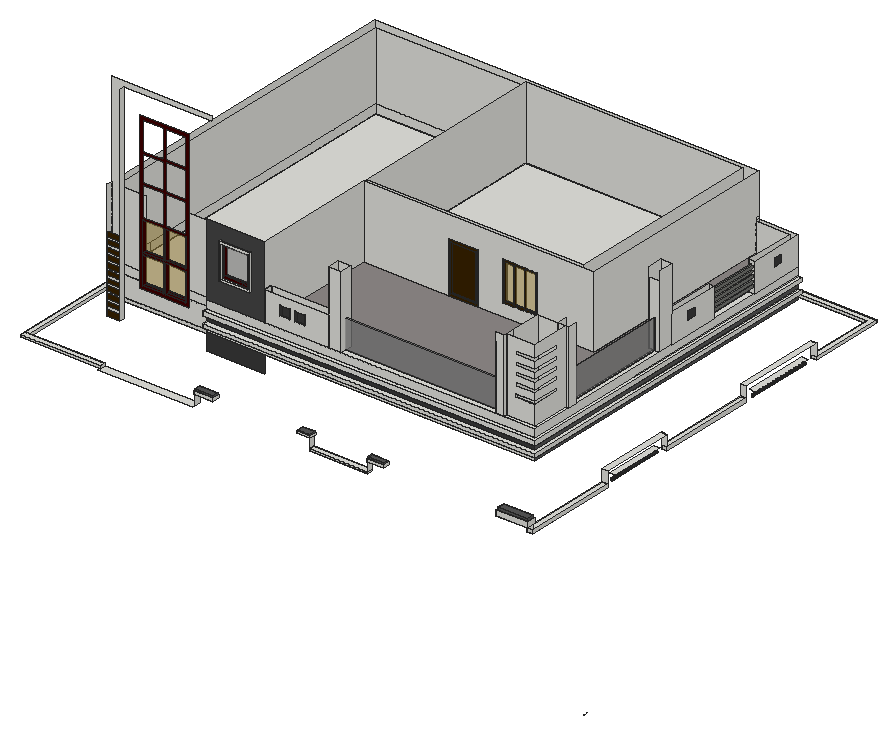
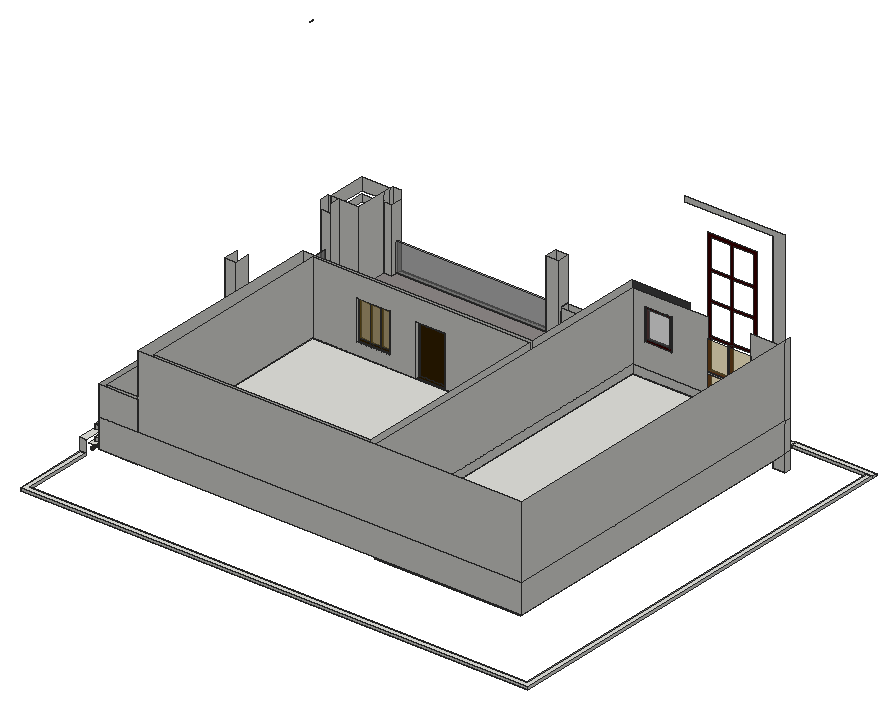
# SketchUp Ruby script. Lengths in inches.
U = 1.inch
M = Sketchup.active_model
def pt(a) = Geom::Point3d.new(a.map { |v| v * U })
def face(e, loops, mat)
  f = e.add_face(loops[0].map { |a| pt(a) })
  loops[1..].each { |l| e.add_face(l.map { |a| pt(a) }).erase! }
  f.material = f.back_material = mat if mat
  f
end
# faces: each face lists its corners as indices into pts; further lists are holes
def faces(e, pts, list, mat = nil) = list.each { |f| face(e, (f[0].is_a?(Array) ? f : [f]).map { |l| l.map { |i| pts[i] } }, mat) }
# xy, xz, yz: faces in a plane at the given z, y or x. An outline is a flat list of corners, or four numbers for a rectangle; further outlines are holes
def ring(l) = l.size == 4 ? [[l[0], l[1]], [l[2], l[1]], [l[2], l[3]], [l[0], l[3]]] : l.each_slice(2).to_a
def flat(e, list, mat, &to3) = list.each { |f| face(e, (f[0].is_a?(Array) ? f : [f]).map { |l| ring(l).map { |u, v| to3.(u, v) } }, mat) }
def xy(e, z, list, mat = nil) = flat(e, list, mat) { |x, y| [x, y, z] }
def xz(e, y, list, mat = nil) = flat(e, list, mat) { |x, z| [x, y, z] }
def yz(e, x, list, mat = nil) = flat(e, list, mat) { |y, z| [x, y, z] }
def lines(e, pts, list) = list.each { |a, b| e.add_line(pt(pts[a]), pt(pts[b])) }
# prism: a flat outline (further loops are holes) pulled along v
def prism(e, loops, v, mat = nil)
  f = face(e, loops, mat); d = Geom::Vector3d.new(v.map { |x| x * U })
  f.pushpull(f.normal.samedirection?(d) ? d.length : -d.length)
end
def box(e, o, s, mat = nil) = prism(e, [[o, [o[0] + s[0], o[1], o[2]], [o[0] + s[0], o[1] + s[1], o[2]], [o[0], o[1] + s[1], o[2]]]], [0, 0, s[2]], mat)
def at(x, y, z, deg = 0) = Geom::Transformation.translation(pt([x, y, z])) * Geom::Transformation.rotation(ORIGIN, Z_AXIS, deg.degrees)
def axes(o, x, y, z) = Geom::Transformation.new([*x, 0, *y, 0, *z, 0, *pt(o).to_a, 1])
def part(name) = M.definitions.add(name)
# library, detail: a bought-in or finely detailed component or shape, given as its bounding box
def library(name, o, s) = part(name).tap { |d| box(d.entities, o, s) }
def detail(e, o, s) = box(e.add_group.entities, o, s)
def put(e, d, t, mat = nil) = e.add_instance(d, t).tap { |i| i.material = mat if mat }
def group(e, t, mat = nil) = e.add_group.tap { |g| g.transformation = t; g.material = mat if mat }.entities
root = M.entities
M.materials.add("[Color A08]").color = [56, 34, 0]
M.materials.add("[Color A08]1").color = [63, 0, 0]
M.materials.add("[Color M06]").color = [86, 86, 86]
M.materials.add("[Color M07]").color = [58, 58, 58]
M.materials.add("[Color M08]").color = [30, 30, 30]
M.materials.add("[Granite Dark Gray]").color = [69, 68, 68]
M.materials.add("[Metal Seamed]1").color = [118, 119, 115]
M.materials.add("[Stone Marble]").color = [143, 138, 136]
M.materials.add("[Translucent Glass Blue]").color = [179, 149, 61]
M.materials["[Translucent Glass Blue]"].alpha = 0.5
M.materials.add("[Translucent Glass Gray]").color = [128, 128, 128]
M.materials["[Translucent Glass Gray]"].alpha = 0.5
c1 = part("Group\#1")
xy(c1.entities,0,[[0,0,48,2.75]],"[Color A08]")
xy(c1.entities,3.37,[[3.37,0,44.63,2.75]],"[Color A08]")
xy(c1.entities,80.63,[[3.37,0,44.63,2.75]],"[Color A08]")
xy(c1.entities,84,[[0,0,48,2.75]],"[Color A08]")
xz(c1.entities,0,[[[0,0,48,84],[3.37,3.37,44.63,80.63]]],"[Color A08]")
xz(c1.entities,2.75,[[[0,0,48,84],[3.37,3.37,44.63,80.63]],[3.37,3.37,44.63,80.63]],"[Color A08]")
yz(c1.entities,0,[[0,0,2.75,84]],"[Color A08]")
yz(c1.entities,3.37,[[0,3.37,2.75,80.63]],"[Color A08]")
yz(c1.entities,44.63,[[0,3.37,2.75,80.63]],"[Color A08]")
yz(c1.entities,48,[[0,0,2.75,84]],"[Color A08]")
c2 = part("Group\#2")
xy(c2.entities,0,[[0,0,80.25,5.625]],"[Color A08]")
xy(c2.entities,3.1,[[3.1,0,25.78,5.625],[27.03,0,50.28,5.625],[51.53,0,77.15,5.625]],"[Color A08]")
xy(c2.entities,66.65,[[3.1,0,25.78,5.625],[27.03,0,50.28,5.625],[51.53,0,77.15,5.625]],"[Color A08]")
xy(c2.entities,69.75,[[0,0,80.25,5.625]],"[Color A08]")
xz(c2.entities,0,[[[0,0,80.25,69.75],[51.53,3.1,77.15,66.65],[27.03,3.1,50.28,66.65],[3.1,3.1,25.78,66.65]]],"[Color A08]")
xz(c2.entities,5.625,[[[0,0,80.25,69.75],[51.53,3.1,77.15,66.65],[27.03,3.1,50.28,66.65],[3.1,3.1,25.78,66.65]]],"[Color A08]")
xz(c2.entities,5.625,[[3.1,3.1,25.78,66.65],[27.03,3.1,50.28,66.65],[51.53,3.1,77.15,66.65]],"[Translucent Glass Blue]")
yz(c2.entities,0,[[0,0,5.625,69.75]],"[Color A08]")
yz(c2.entities,3.1,[[0,3.1,5.625,66.65]],"[Color A08]")
yz(c2.entities,25.78,[[0,3.1,5.625,66.65]],"[Color A08]")
yz(c2.entities,27.03,[[0,3.1,5.625,66.65]],"[Color A08]")
yz(c2.entities,50.28,[[0,3.1,5.625,66.65]],"[Color A08]")
yz(c2.entities,51.53,[[0,3.1,5.625,66.65]],"[Color A08]")
yz(c2.entities,77.15,[[0,3.1,5.625,66.65]],"[Color A08]")
yz(c2.entities,80.25,[[0,0,5.625,69.75]],"[Color A08]")
prism(root,[[[834.64,582.45,107.43],[835.13,582.45,107.31],[835.64,582.45,107.32],[836.12,582.45,107.46],[836.55,582.45,107.73],[836.9,582.45,108.09],[837.14,582.45,108.54],[837.26,582.45,109.03],[837.25,582.45,109.53],[837.11,582.45,110.02],[836.85,582.45,110.45],[836.48,582.45,110.8],[836.04,582.45,111.04],[835.55,582.45,111.16],[835.04,582.45,111.15],[834.55,582.45,111.01],[834.12,582.45,110.74],[833.77,582.45,110.38],[833.53,582.45,109.93],[833.41,582.45,109.44],[833.42,582.45,108.9375],[833.57,582.45,108.45],[833.83,582.45,108.02],[834.19,582.45,107.67]]],[0,91.75,0],"[Color M07]")
xy(root,105,[[132.5,398.15,288.93,411.9],[0,402.9,132.5,411.9],[478.28,402.9,575.03,411.9],[0,411.9,0,1122.9,840,1122.9,840,999.11,831,999.11,831,1113.9,9,1113.9,9,411.9],[831,411.9,840,566.77],
  [831,690.36,840,853.98]])
xy(root,107.75,[[478.28,402.9,575.03,411.9]])
xy(root,109,[[0,402.9,132.5,411.9],[0,411.9,9,411.9,9,1113.9,831,1113.9,831,999.11,840,999.11,840,1122.9,0,1122.9]])
xy(root,110.5,[[831,411.9,840,566.77]])
xy(root,111.25,[[831,690.36,840,853.98]])
xy(root,113.38,[[831,872.22,840,980.28]])
xy(root,117,[[470.84,700.96,518.84,706.96]])
xy(root,117.03,[[831,582.45,840,674.33]])
xy(root,119.375,[[789.41,399.71,789.41,415.09,831,415.09,831,411.9,791.47,411.9,791.47,402.9,840,402.9,840,411.9,831,411.9,831,415.09,841.625,415.09,841.625,399.71]])
xy(root,122.6875,[[[287.74,401.21,319.84,413.9],[288.93,402.9,318.78,411.9]]])
xy(root,122.82,[[560.85,700.96,616.42,706.96]])
xy(root,123,[[791.47,402.9,840,411.9]])
xy(root,123.125,[[[574.09,401.34,602.04,413.34],[575.03,402.9,600.6,411.9]]])
xy(root,124.5625,[[288.93,402.9,318.78,411.9]])
xy(root,124.6875,[[[458.12,401.02,479.97,413.09],[459.31,402.9,478.28,411.9]]])
xy(root,124.8125,[[575.03,402.9,600.6,411.9]])
xy(root,125.23,[[75.5,487.84,96.69,496.71]])
xy(root,125.4375,[[459.31,402.9,478.28,411.9]])
xy(root,127.5625,[[[789.41,399.71,841.625,415.09],[791.47,401.77,840,413.15]],[[458.12,401.02,479.97,413.09],[458.93,402.02,479.22,412.65]],[[287.74,401.21,319.84,413.9],[288.43,402.46,318.78,412.77]],[[574.09,401.34,602.04,413.34],[575.03,402.59,600.85,411.96]],[791.47,401.77,840,413.15],
  [458.93,402.02,479.22,412.65],[288.43,402.46,318.78,412.77],[575.03,402.59,600.85,411.96]])
xy(root,129.375,[[575.03,402.59,600.85,411.96]],"[Color M06]")
xy(root,129.5,[[831,566.77,840,690.36],[831,853.98,840,999.11]])
xy(root,129.5,[[458.93,402.02,479.22,412.65]],"[Color M06]")
xy(root,130,[[288.43,402.46,318.78,412.77]],"[Color M06]")
xy(root,131.6875,[[791.47,401.77,840,413.15]],"[Color M06]")
xy(root,147,[[81.5,502.71,323.75,1035.15]])
xy(root,153,[[329.75,496.71,329.75,700.96,710.3125,700.96,710.3125,1041.15,776.3125,1041.15,776.3125,496.71],[81.5,502.71,323.75,1035.15]])
xy(root,163.0625,[[233.4,489.27,329.75,496.71],[329.75,489.27,782.0625,496.71],[329.75,496.71,776.3125,700.96],[776.3125,496.71,782.0625,1041.09]])
xy(root,163.22,[[1254.01,0,1254.88,6]],"[Color M08]")
xy(root,169.125,[[233.4,489.27,782.0625,489.27,782.0625,1041.09,776.3125,1041.09,776.3125,496.71,233.4,496.71],[329.75,496.71,776.3125,700.96]])
xy(root,180.8125,[[233.4,489.27,329.75,496.71],[329.75,489.27,782.0625,496.71],[329.75,496.71,776.3125,700.96],[776.3125,496.71,782.0625,1041.15]])
xy(root,184.79,[[128.05,496.71,161.69,502.71],[165.04,496.71,198.99,502.71]],"[Color A08]1")
xy(root,187,[[81.5,502.71,323.75,1035.15]])
xy(root,187.875,[[233.4,489.27,782.0625,489.27,782.0625,1041.15,776.3125,1041.15,776.3125,496.71,233.4,496.71],[329.75,496.71,776.3125,700.96]])
xy(root,195,[[329.75,706.96,689.4375,1035.15]])
xy(root,201,[[329.75,496.71,434.48,511.31],[434.48,496.71,455.35,516.84],[455.35,496.71,712.1,504.34],[712.1,496.71,724.73,514.59],[724.73,496.71,776.3125,502.4],
  [724.73,502.4,771.75,566.61],[771.75,502.4,776.3125,566.61],[455.35,504.34,712.1,506.34],[758.97,566.61,776.3125,581.49],[767.0625,581.49,769.0625,754.59],
  [769.0625,581.49,776.3125,754.59],[329.75,706.96,689.4375,1035.15],[689.4375,706.96,710.3125,1035.15],[758.0625,754.59,776.3125,780.03],[767.1875,780.03,776.3125,867.13],
  [767.1875,867.13,776.3125,951.14],[767.1875,951.14,767.1875,1035.15,710.3125,1035.15,710.3125,1041.15,776.3125,1041.15,776.3125,951.14]])
xy(root,201,[[455.35,506.34,712.1,506.34,712.1,514.59,724.73,514.59,724.73,566.61,758.97,566.61,758.97,581.49,767.0625,581.49,767.0625,754.59,758.0625,754.59,758.0625,780.03,767.1875,780.03,767.1875,1035.15,710.3125,1035.15,710.3125,700.96,518.51,700.96,518.51,706.96,470.51,706.96,470.51,700.96,329.75,700.96,329.75,511.31,434.48,511.31,434.48,516.84,455.35,516.84]],"[Stone Marble]")
xy(root,208.99,[[769.27,867.13,773.7,951.14]],"[Metal Seamed]1")
xy(root,212.93,[[769.27,867.13,773.7,951.14]],"[Metal Seamed]1")
xy(root,216.37,[[769.27,867.13,773.7,952.63]],"[Metal Seamed]1")
xy(root,219.98,[[354.55,496.71,370.43,499.46],[379.61,496.71,395.49,499.46]],"[Color M07]")
xy(root,220.31,[[769.27,867.13,773.7,952.63]],"[Metal Seamed]1")
xy(root,221.54,[[773.75,811.33,776.3125,829.45],[773.3125,989.77,776.3125,1007.89]],"[Color M07]")
xy(root,221.63,[[560.85,700.96,616.42,706.96]])
xy(root,223.74,[[769.27,867.13,773.7,951.14]],"[Metal Seamed]1")
xy(root,227.68,[[769.27,867.13,773.7,951.14]],"[Metal Seamed]1")
xy(root,231.09,[[128.05,496.71,161.69,502.71],[165.04,496.71,198.99,502.71]],"[Color A08]1")
xy(root,231.12,[[769.27,867.13,773.7,953.26]],"[Metal Seamed]1")
xy(root,232.42,[[739.88,502.4,771.75,502.4,771.75,547.34,770.3125,547.34,770.3125,504.4,739.88,504.4]])
xy(root,234.11,[[128.05,496.71,161.69,502.71],[165.04,496.71,198.99,502.71]],"[Color A08]1")
xy(root,235.06,[[769.27,867.13,773.7,953.26]],"[Metal Seamed]1")
xy(root,235.85,[[354.55,496.71,370.43,499.46],[379.61,496.71,395.49,499.46]],"[Color M07]")
xy(root,236.86,[[773.75,811.33,776.3125,829.45],[773.3125,989.77,776.3125,1007.89]],"[Color M07]")
xy(root,237.79,[[739.88,502.4,745.57,504.4],[745.57,502.4,771.75,504.4],[770.3125,504.4,771.75,547.34]])
xy(root,238.49,[[769.27,867.13,773.7,951.82]],"[Metal Seamed]1")
xy(root,238.6875,[[255.94,493.59,306.57,496.71]])
xy(root,241.34,[[258.89,493.59,303.7,502.71]])
xy(root,242.43,[[769.27,867.13,773.7,951.82]],"[Metal Seamed]1")
xz(root,399.71,[[789.41,119.375,841.625,127.5625]])
xz(root,401.02,[[458.12,124.6875,479.97,127.5625]])
xz(root,401.21,[[287.74,122.6875,319.84,127.5625]])
xz(root,401.34,[[574.09,123.125,602.04,127.5625]])
xz(root,401.77,[[791.47,127.5625,840,131.6875]],"[Color M06]")
xz(root,402.02,[[458.93,127.5625,479.22,129.5]],"[Color M06]")
xz(root,402.46,[[288.43,127.5625,318.78,130]],"[Color M06]")
xz(root,402.59,[[575.03,127.5625,600.85,129.375]],"[Color M06]")
xz(root,402.9,[[0,105,132.5,109],[478.28,105,575.03,107.75],[791.47,119.375,840,123],[288.93,122.6875,318.78,124.5625],[575.03,123.125,600.6,124.8125],
  [459.31,124.6875,478.28,125.4375]])
xz(root,411.9,[[0,105,9,109],[9,105,132.5,109],[478.28,105,575.03,107.75],[831,105,840,110.5],[831,110.5,840,119.375],
  [791.47,119.375,831,123],[831,119.375,840,123],[288.93,122.6875,318.78,124.5625],[575.03,123.125,600.6,124.8125],[459.31,124.6875,478.28,125.4375]])
xz(root,411.96,[[575.03,127.5625,600.85,129.375]],"[Color M06]")
xz(root,412.65,[[458.93,127.5625,479.22,129.5]],"[Color M06]")
xz(root,412.77,[[288.43,127.5625,318.78,130]],"[Color M06]")
xz(root,413.09,[[458.12,124.6875,479.97,127.5625]])
xz(root,413.15,[[791.47,127.5625,840,131.6875]],"[Color M06]")
xz(root,413.34,[[574.09,123.125,602.04,127.5625]])
xz(root,413.9,[[287.74,122.6875,319.84,127.5625]])
xz(root,415.09,[[789.41,119.375,841.625,127.5625]])
xz(root,487.84,[[75.5,136.53,96.69,139.83],[75.5,148.03,96.69,151.33],[75.5,159.53,96.69,162.83],[75.5,171.03,96.69,174.33],[75.5,182.53,96.69,185.83],
  [75.5,194.03,96.69,197.33],[75.5,205.53,96.69,208.83],[75.5,217.03,96.69,220.33],[75.5,228.53,96.69,231.83],[75.5,240.03,96.69,243.33]])
xz(root,487.84,[[75.5,125.23,96.69,136.53],[75.5,139.83,96.69,148.03],[75.5,151.33,96.69,159.53],[75.5,162.83,96.69,171.03],[75.5,174.33,96.69,182.53],
  [75.5,185.83,96.69,194.03],[75.5,197.33,96.69,205.53],[75.5,208.83,96.69,217.03],[75.5,220.33,96.69,228.53],[75.5,231.83,96.69,240.03],
  [75.5,243.33,96.69,251.53]],"[Color A08]")
xz(root,489.27,[[233.4,163.0625,782.0625,169.125],[233.4,180.8125,782.0625,187.875]])
xz(root,493.59,[[[255.94,238.6875,306.57,297.5625],[258.89,241.34,303.7,294.03]]])
xz(root,496.71,[[75.5,125.23,75.5,477,241.19,477,241.19,468.42,96.69,468.42,96.69,125.23],[233.4,153,776.3125,163.0625],[233.4,187.875,776.3125,201],[[329.75,201,434.48,249],[354.55,219.98,370.43,235.85],[379.61,219.98,395.49,235.85]],[434.48,201,455.35,321],
  [712.1,201,724.73,321]])
xz(root,496.71,[[[122.69,179.43,204.35,436.03],[165.04,284.92,198.99,334.65],[128.05,284.92,161.69,334.65],[165.04,234.11,198.99,281.9],[128.05,234.11,161.69,281.9],[165.04,383.86,198.99,430.67],[128.05,383.86,161.69,430.67],[165.04,184.79,198.99,231.09],[128.05,184.79,161.69,231.09],[165.04,337.67,198.99,380.84],[128.05,337.67,161.69,380.84]]],"[Color A08]1")
xz(root,496.71,[[233.4,125.23,329.75,153],[233.4,169.125,776.3125,180.8125]],"[Color M07]")
xz(root,496.71,[[[233.4,201,329.75,321],[255.94,238.6875,306.57,297.5625]]],"[Granite Dark Gray]")
xz(root,499.46,[[354.55,219.98,370.43,235.85],[379.61,219.98,395.49,235.85]],"[Color M07]")
xz(root,502.4,[[724.73,201,771.75,201,771.75,232.42,739.88,232.42,739.88,237.79,771.75,237.79,771.75,249.35,739.88,249.35,739.88,254.73,771.75,254.73,771.75,264.67,739.88,264.67,739.88,270.04,771.75,270.04,771.75,279.42,739.88,279.42,739.88,284.79,771.75,284.79,771.75,295.73,739.88,295.73,739.88,301.1,771.75,301.1,771.75,321,724.73,321]])
xz(root,502.71,[[81.5,147,323.75,153],[81.5,153,81.5,187,128.05,187,128.05,184.79,198.99,184.79,198.99,187,323.75,187,323.75,153],[161.69,184.79,165.04,187],[81.5,187,128.05,201],[161.69,187,165.04,231.09],
  [198.99,187,323.75,201],[81.5,201,128.05,315],[[198.99,201,323.75,315],[258.89,241.34,303.7,294.03]],[128.05,231.09,161.69,234.11],[161.69,231.09,165.04,234.11],
  [165.04,231.09,198.99,234.11],[161.69,234.11,165.04,281.9]])
xz(root,502.71,[[128.05,184.79,161.69,187],[165.04,184.79,198.99,187]],"[Color A08]1")
xz(root,502.71,[[128.05,187,161.69,231.09],[165.04,187,198.99,231.09],[128.05,234.11,161.69,281.9],[165.04,234.11,198.99,281.9]],"[Translucent Glass Blue]")
xz(root,504.34,[[455.35,201,712.1,249]],"[Translucent Glass Gray]")
xz(root,504.4,[[739.88,232.42,770.3125,237.79]])
xz(root,506.34,[[455.35,201,712.1,249]],"[Translucent Glass Gray]")
xz(root,511.31,[[329.75,201,434.48,249]])
xz(root,514.59,[[712.1,201,724.73,306.3125]])
xz(root,516.84,[[434.48,201,455.35,321]])
xz(root,547.34,[[770.3125,232.42,771.75,237.79]])
xz(root,566.61,[[724.73,201,758.97,321],[758.97,201,771.75,321],[771.75,201,776.3125,321]])
xz(root,566.77,[[831,105,840,110.5],[831,110.5,840,129.5]])
xz(root,581.49,[[758.97,201,758.97,306.3125,776.3125,306.3125,776.3125,201,769.0625,201,769.0625,256.0625,767.0625,256.0625,767.0625,201],[767.0625,201,769.0625,249]])
xz(root,690.36,[[831,105,840,111.25],[831,111.25,840,129.5]])
xz(root,700.96,[[329.75,163.0625,776.3125,169.125],[329.75,180.8125,776.3125,187.875],[[329.75,201,470.51,201,470.51,285,518.51,285,518.51,201,710.3125,201,710.3125,321,329.75,321],[560.85,221.63,616.42,286.38]]])
xz(root,706.96,[[329.75,153,689.4375,195],[329.75,195,351.94,201],[351.94,195,400.13,201],[400.13,195,470.51,201],[470.51,195,518.51,201],
  [518.51,195,689.4375,201],[[329.75,201,329.75,321,689.4375,321,689.4375,201,518.51,201,518.51,285,470.51,285,470.51,201],[560.85,221.63,616.42,286.38]]])
xz(root,754.59,[[758.0625,201,767.0625,201,767.0625,256.0625,769.0625,256.0625,769.0625,201,776.3125,201,776.3125,306.3125,758.0625,306.3125],[767.0625,201,769.0625,249]])
xz(root,780.03,[[758.0625,201,758.0625,321,776.3125,321,776.3125,252.0625,767.1875,252.0625,767.1875,201],[767.1875,201,776.3125,249]])
xz(root,811.33,[[773.75,221.54,776.3125,236.86]],"[Color M07]")
xz(root,829.45,[[773.75,221.54,776.3125,236.86]],"[Color M07]")
xz(root,853.98,[[831,105,840,111.25],[831,111.25,840,129.5]])
xz(root,867.13,[[[767.1875,201,776.3125,249],[769.27,238.49,773.7,242.43],[769.27,231.12,773.7,235.06],[769.27,223.74,773.7,227.68],[769.27,216.37,773.7,220.31],[769.27,208.99,773.7,212.93]]])
xz(root,867.13,[[769.27,208.99,773.7,212.93],[769.27,216.37,773.7,220.31],[769.27,223.74,773.7,227.68],[769.27,231.12,773.7,235.06],[769.27,238.49,773.7,242.43]],"[Metal Seamed]1")
xz(root,872.22,[[835.68,104.38,836.15,104.43,836.59,104.61,836.97,104.89,837.27,105.26,837.45,105.69,837.53,106.16,837.47,106.63,837.3,107.07,837.02,107.45,836.65,107.74,836.21,107.93,835.75,108,835.28,107.95,834.84,107.78,834.46,107.5,834.16,107.13,833.97,106.69,833.9,106.23,833.95,105.76,834.125,105.32,834.41,104.93,834.78,104.64,835.21,104.45]],"[Color M07]")
xz(root,951.14,[[[767.1875,201,776.3125,249],[769.27,208.99,773.7,212.93],[769.27,223.74,773.7,227.68]]])
xz(root,951.82,[[769.27,238.49,773.7,242.43]],"[Metal Seamed]1")
xz(root,952.63,[[769.27,216.37,773.7,220.31]],"[Metal Seamed]1")
xz(root,953.26,[[769.27,231.12,773.7,235.06]],"[Metal Seamed]1")
xz(root,989.77,[[773.3125,221.54,776.3125,236.86]],"[Color M07]")
xz(root,999.11,[[831,105,840,109],[831,109,840,129.5]])
xz(root,1007.89,[[773.3125,221.54,776.3125,236.86]],"[Color M07]")
xz(root,1035.15,[[81.5,147,323.75,153],[81.5,153,323.75,187],[329.75,153,689.4375,195],[81.5,187,323.75,201],[329.75,195,689.4375,201],
  [81.5,201,323.75,315],[329.75,201,689.4375,321],[710.3125,201,767.1875,249]])
xz(root,1041.09,[[776.3125,163.0625,782.0625,169.125]])
xz(root,1041.15,[[75.5,153,776.3125,201],[776.3125,180.8125,782.0625,187.875],[75.5,201,710.3125,321],[710.3125,201,776.3125,249]])
xz(root,1113.9,[[9,105,831,109]])
xz(root,1122.9,[[0,105,840,109]])
yz(root,0,[[402.9,105,411.9,109],[411.9,105,1122.9,109]])
yz(root,9,[[411.9,105,1113.9,109]])
yz(root,75.5,[[487.84,125.23,496.71,153],[487.84,153,496.71,201],[496.71,153,1041.15,201],[487.84,201,496.71,321],[496.71,201,1041.15,321]])
yz(root,81.5,[[502.71,147,1035.15,153],[502.71,153,1035.15,187],[502.71,187,568.94,201],[568.94,187,608.76,201],[608.76,187,1035.15,201],
  [502.71,201,1035.15,315]])
yz(root,96.69,[[487.84,125.23,496.71,468.42]])
yz(root,128.05,[[496.71,184.79,502.71,231.09],[496.71,234.11,502.71,281.9]],"[Color A08]1")
yz(root,132.5,[[402.9,105,411.9,109]])
yz(root,161.69,[[496.71,184.79,502.71,231.09],[496.71,234.11,502.71,281.9]],"[Color A08]1")
yz(root,165.04,[[496.71,184.79,502.71,231.09],[496.71,234.11,502.71,281.9]],"[Color A08]1")
yz(root,198.99,[[496.71,184.79,502.71,231.09],[496.71,234.11,502.71,281.9]],"[Color A08]1")
yz(root,233.4,[[489.27,163.0625,496.71,169.125],[489.27,180.8125,496.71,187.875]])
yz(root,255.94,[[493.59,238.6875,496.71,297.5625]])
yz(root,258.89,[[493.59,241.34,502.71,294.03]])
yz(root,287.74,[[401.21,122.6875,413.9,127.5625]])
yz(root,288.43,[[402.46,127.5625,412.77,130]],"[Color M06]")
yz(root,288.93,[[402.9,105,411.9,122.6875],[402.9,122.6875,411.9,124.5625]])
yz(root,303.7,[[493.59,241.34,502.71,294.03]])
yz(root,306.57,[[493.59,238.6875,496.71,297.5625]])
yz(root,318.78,[[402.9,122.6875,411.9,124.5625]])
yz(root,318.78,[[402.46,127.5625,412.77,130]],"[Color M06]")
yz(root,319.84,[[401.21,122.6875,413.9,127.5625]])
yz(root,323.75,[[502.71,147,1035.15,153],[502.71,153,1035.15,187],[502.71,187,1035.15,201],[502.71,201,1035.15,315]])
yz(root,329.75,[[706.96,153,1035.15,195],[706.96,195,1035.15,201],[496.71,201,511.31,249],[511.31,201,700.96,201,700.96,321,496.71,321,496.71,251.5625,511.31,251.5625],[706.96,201,1035.15,321]])
yz(root,354.55,[[496.71,219.98,499.46,235.85]],"[Color M07]")
yz(root,370.43,[[496.71,219.98,499.46,235.85]],"[Color M07]")
yz(root,379.61,[[496.71,219.98,499.46,235.85]],"[Color M07]")
yz(root,395.49,[[496.71,219.98,499.46,235.85]],"[Color M07]")
yz(root,434.48,[[496.71,201,511.31,249],[511.31,201,511.31,251.5625,496.71,251.5625,496.71,321,516.84,321,516.84,201]])
yz(root,455.35,[[496.71,201,504.34,201,504.34,253.3125,506.34,253.3125,506.34,201,516.84,201,516.84,321,496.71,321],[504.34,201,506.34,249]])
yz(root,458.12,[[401.02,124.6875,413.09,127.5625]])
yz(root,458.93,[[402.02,127.5625,412.65,129.5]],"[Color M06]")
yz(root,459.31,[[402.9,124.6875,411.9,125.4375]])
yz(root,470.51,[[700.96,201,706.96,285]])
yz(root,478.28,[[402.9,105,411.9,107.75],[402.9,107.75,411.9,124.6875],[402.9,124.6875,411.9,125.4375]])
yz(root,479.22,[[402.02,127.5625,412.65,129.5]],"[Color M06]")
yz(root,479.97,[[401.02,124.6875,413.09,127.5625]])
yz(root,518.51,[[700.96,201,706.96,285]])
yz(root,560.85,[[700.96,221.63,706.96,286.38]])
yz(root,574.09,[[401.34,123.125,413.34,127.5625]])
yz(root,575.03,[[402.9,105,411.9,107.75],[402.9,107.75,411.9,123.125],[402.9,123.125,411.9,124.8125]])
yz(root,575.03,[[402.59,127.5625,411.96,129.375]],"[Color M06]")
yz(root,600.6,[[402.9,123.125,411.9,124.8125]])
yz(root,600.85,[[402.59,127.5625,411.96,129.375]],"[Color M06]")
yz(root,602.04,[[401.34,123.125,413.34,127.5625]])
yz(root,616.42,[[700.96,221.63,706.96,286.38]])
yz(root,689.4375,[[706.96,153,1035.15,195],[706.96,195,1035.15,201],[706.96,201,1035.15,321]])
yz(root,710.3125,[[700.96,201,1035.15,201,1035.15,253.6875,1041.15,253.6875,1041.15,321,700.96,321],[1035.15,201,1041.15,249]])
yz(root,712.1,[[496.71,201,496.71,306.3125,514.59,306.3125,514.59,201,506.34,201,506.34,253.3125,504.34,253.3125,504.34,201],[504.34,201,506.34,249]])
yz(root,724.73,[[496.71,201,502.4,321],[502.4,201,514.59,321],[514.59,201,514.59,306.3125,515.78,306.3125,515.78,321,566.61,321,566.61,201]])
yz(root,739.88,[[502.4,232.42,504.4,237.79]])
yz(root,758.0625,[[754.59,201,780.03,321]])
yz(root,758.97,[[566.61,201,581.49,321]])
yz(root,767.0625,[[581.49,201,754.59,249]],"[Translucent Glass Gray]")
yz(root,767.1875,[[780.03,201,867.13,249],[951.14,201,1035.15,249]])
yz(root,769.0625,[[581.49,201,754.59,249]],"[Translucent Glass Gray]")
yz(root,769.27,[[867.13,208.99,951.14,212.93],[867.13,216.37,952.63,220.31],[867.13,223.74,951.14,227.68],[867.13,231.12,953.26,235.06],[867.13,238.49,951.82,242.43]],"[Metal Seamed]1")
yz(root,770.3125,[[504.4,232.42,547.34,237.79]])
yz(root,771.75,[[502.4,201,566.61,201,566.61,321,502.4,321,502.4,301.1,547.34,301.1,547.34,295.73,502.4,295.73,502.4,284.79,547.34,284.79,547.34,279.42,502.4,279.42,502.4,270.04,547.34,270.04,547.34,264.67,502.4,264.67,502.4,254.73,547.34,254.73,547.34,249.35,502.4,249.35,502.4,237.79,547.34,237.79,547.34,232.42,502.4,232.42]])
yz(root,773.3125,[[989.77,221.54,1007.89,236.86]],"[Color M07]")
yz(root,773.7,[[867.13,208.99,951.14,212.93],[867.13,216.37,952.63,220.31],[867.13,223.74,951.14,227.68],[867.13,231.12,953.26,235.06],[867.13,238.49,951.82,242.43]],"[Metal Seamed]1")
yz(root,773.75,[[811.33,221.54,829.45,236.86]],"[Color M07]")
yz(root,776.3125,[[700.96,163.0625,1041.09,169.125],[700.96,180.8125,1041.15,187.875],[496.71,187.875,1041.15,201],[566.61,201,581.49,321],[754.59,201,780.03,321],
  [[780.03,201,867.13,249],[811.33,221.54,829.45,236.86]],[[951.14,201,1041.15,249],[989.77,221.54,1007.89,236.86]]])
yz(root,776.3125,[[496.71,153,1041.15,153,1041.15,180.8125,496.71,180.8125,496.71,169.125,1041.09,169.125,1041.09,163.0625,496.71,163.0625]],"[Color M06]")
yz(root,782.0625,[[489.27,163.0625,1041.09,169.125],[489.27,180.8125,1041.15,187.875]])
yz(root,789.41,[[399.71,119.375,415.09,127.5625]])
yz(root,791.47,[[402.9,119.375,411.9,123]])
yz(root,791.47,[[401.77,127.5625,413.15,131.6875]],"[Color M06]")
yz(root,831,[[411.9,105,566.77,110.5],[690.36,105,853.98,111.25],[999.11,105,1113.9,109],[411.9,119.375,415.09,119.375,411.9,123]])
yz(root,840,[[411.9,105,566.77,110.5],[690.36,105,853.98,111.25],[999.11,105,1122.9,109],[402.9,119.375,411.9,123]])
yz(root,840,[[401.77,127.5625,413.15,131.6875]],"[Color M06]")
yz(root,841.625,[[399.71,119.375,415.09,127.5625]])
p = [[835.68,872.22,104.38],[835.21,872.22,104.45],[835.21,980.28,104.45],[835.68,980.28,104.38],[836.15,872.22,104.43],[836.15,980.28,104.43],
  [836.59,872.22,104.61],[836.59,980.28,104.61],[834.78,872.22,104.64],[834.78,980.28,104.64],[834.41,872.22,104.93],[834.41,980.28,104.93],
  [836.97,872.22,104.89],[836.97,980.28,104.89],[834.125,872.22,105.32],[834.125,980.28,105.32],[837.27,872.22,105.26],[837.27,980.28,105.26],
  [833.95,872.22,105.76],[833.95,980.28,105.76],[837.45,872.22,105.69],[837.45,980.28,105.69],[837.53,872.22,106.16],[837.53,980.28,106.16],
  [833.9,872.22,106.23],[833.9,980.28,106.23],[833.97,872.22,106.69],[833.97,980.28,106.69],[837.47,872.22,106.63],[837.47,980.28,106.63],
  [837.3,872.22,107.07],[837.3,980.28,107.07],[834.16,872.22,107.13],[834.16,980.28,107.13],[834.46,872.22,107.5],[834.46,980.28,107.5],
  [837.02,872.22,107.45],[837.02,980.28,107.45],[836.65,872.22,107.74],[836.65,980.28,107.74],[834.84,872.22,107.78],[834.84,980.28,107.78],
  [836.21,872.22,107.93],[836.21,980.28,107.93],[835.28,872.22,107.95],[835.28,980.28,107.95],[835.75,872.22,108],[835.75,980.28,108],
  [329.75,700.96,201],[329.75,700.96,187.875],[329.75,700.96,180.8125],[329.75,700.96,169.125]]
faces(root,p,[[0,1,2,3],[4,0,3,5],[6,4,5,7],[1,8,9,2],[8,10,11,9],[12,6,7,13],[10,14,15,11],[16,12,13,17],
  [14,18,19,15],[20,16,17,21],[22,20,21,23],[18,24,25,19],[24,26,27,25],[28,22,23,29],[30,28,29,31],[26,32,33,27],
  [32,34,35,33],[36,30,31,37],[38,36,37,39],[34,40,41,35],[42,38,39,43],[40,44,45,41],[46,42,43,47],[44,46,47,45]],"[Color M07]")
lines(root,p,[[48,49],[50,51]])
put(root,c1,at(470.51,700.96,201))
put(root,c2,axes([560.3,700.96,221.63],[0.6993,0,0],[0,0.37,0],[0,0,0.92832]))
g1 = group(root,at(258.89,498.15,241.34))
xy(g1,0,[[0,0,44.8125,4.5]],"[Color A08]1")
xy(g1,3.95,[[3.3125,0,41.5,4.5]],"[Color A08]1")
xy(g1,49.49,[[3.3125,0,41.5,4.5]],"[Color A08]1")
xy(g1,53.4375,[[0,0,44.8125,4.5]],"[Color A08]1")
xz(g1,0,[[[0,0,44.8125,53.4375],[3.3125,3.95,41.5,49.49]]],"[Color A08]1")
xz(g1,4.5,[[[0,0,44.8125,53.4375],[3.3125,3.95,41.5,49.49]]],"[Color A08]1")
xz(g1,4.5,[[3.3125,3.95,41.5,49.49]],"[Translucent Glass Gray]")
yz(g1,0,[[0,0,4.5,53.4375]],"[Color A08]1")
yz(g1,3.3125,[[0,3.95,4.5,49.49]],"[Color A08]1")
yz(g1,41.5,[[0,3.95,4.5,49.49]],"[Color A08]1")
yz(g1,44.8125,[[0,0,4.5,53.4375]],"[Color A08]1")
